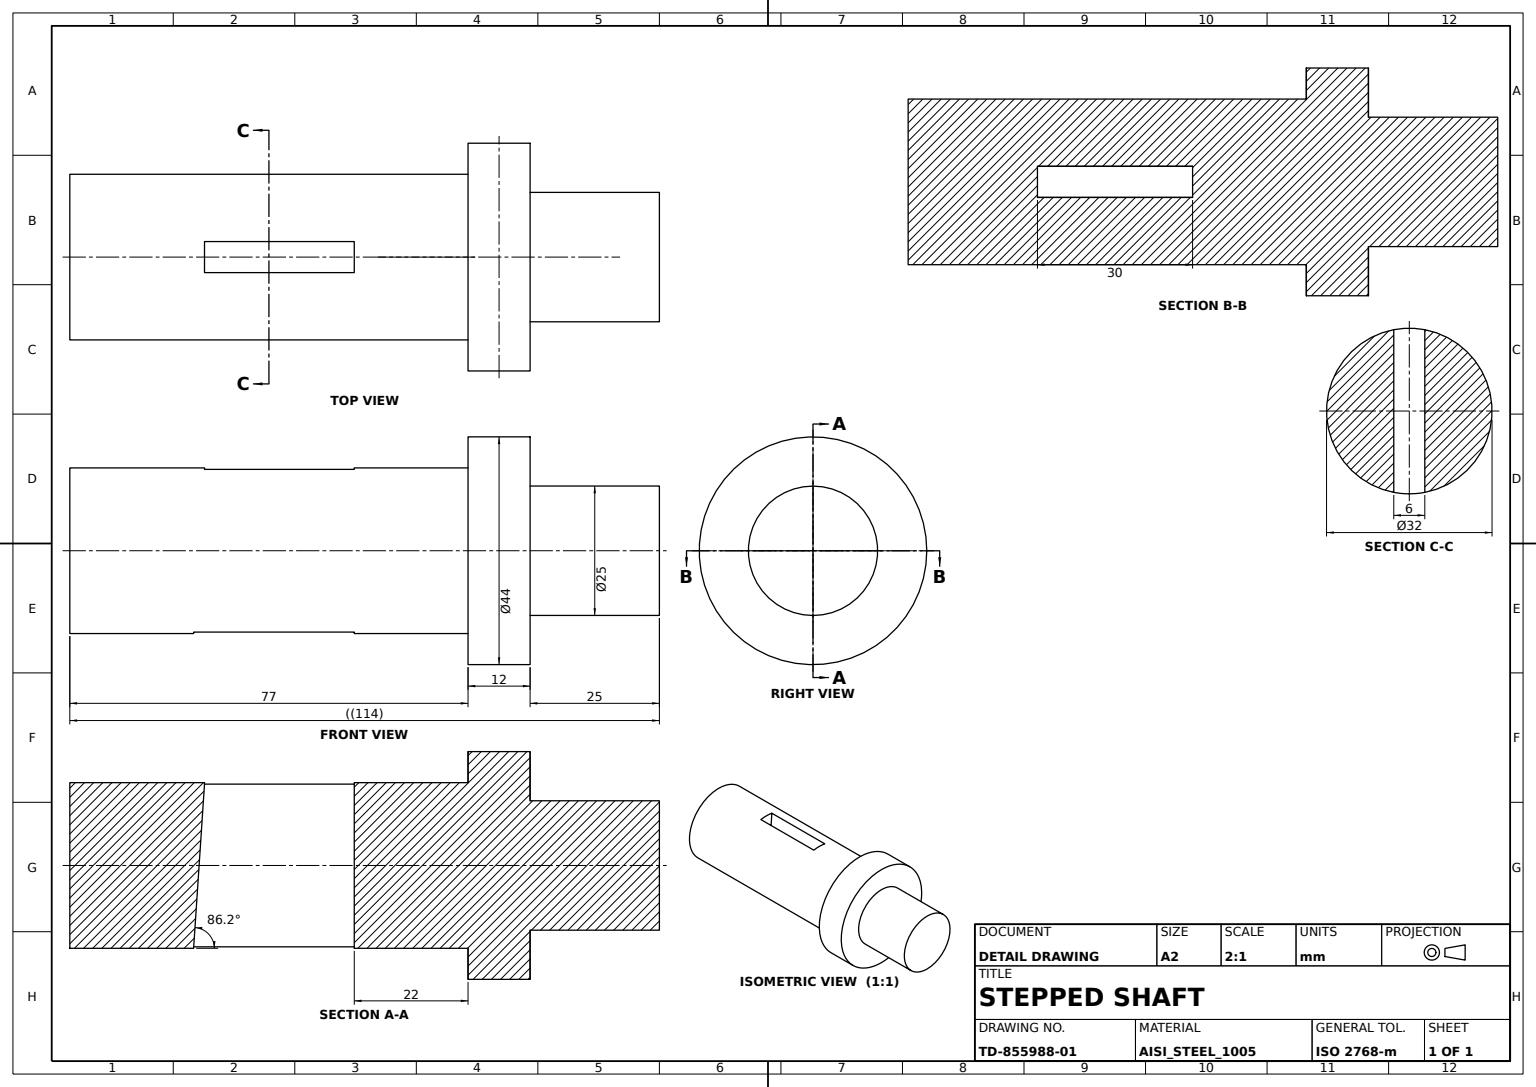
ISO-10303-21;
HEADER;
FILE_DESCRIPTION((''),'2;1');
FILE_NAME('','',(''),(''),'','','');
FILE_SCHEMA(('AUTOMOTIVE_DESIGN'));
ENDSEC;
DATA;
#1=APPLICATION_CONTEXT('');
#2=PRODUCT_CONTEXT('',#1,'mechanical');
#3=PRODUCT('','','',(#2));
#4=PRODUCT_DEFINITION_FORMATION('','',#3);
#5=PRODUCT_DEFINITION_CONTEXT('',#1,'design');
#6=PRODUCT_DEFINITION('','',#4,#5);
#7=PRODUCT_DEFINITION_SHAPE('','',#6);
#8=(LENGTH_UNIT()NAMED_UNIT(*)SI_UNIT(.MILLI.,.METRE.));
#9=(NAMED_UNIT(*)PLANE_ANGLE_UNIT()SI_UNIT($,.RADIAN.));
#10=(NAMED_UNIT(*)SI_UNIT($,.STERADIAN.)SOLID_ANGLE_UNIT());
#11=UNCERTAINTY_MEASURE_WITH_UNIT(LENGTH_MEASURE(0.005),#8,'distance_accuracy_value','');
#12=(GEOMETRIC_REPRESENTATION_CONTEXT(3)GLOBAL_UNCERTAINTY_ASSIGNED_CONTEXT((#11))GLOBAL_UNIT_ASSIGNED_CONTEXT((#8,#9,#10))REPRESENTATION_CONTEXT('',''));
#13=CARTESIAN_POINT('',(16.,0.,-77.));
#14=VERTEX_POINT('',#13);
#15=CARTESIAN_POINT('',(0.,0.,-77.));
#16=DIRECTION('',(0.,0.,-1.));
#17=DIRECTION('',(1.,0.,0.));
#18=AXIS2_PLACEMENT_3D('',#15,#16,#17);
#19=CIRCLE('',#18,16.);
#20=EDGE_CURVE('',#14,#14,#19,.T.);
#21=ORIENTED_EDGE('',*,*,#20,.T.);
#22=EDGE_LOOP('',(#21));
#23=FACE_BOUND('',#22,.T.);
#24=DIRECTION('',(-1.,0.,0.));
#25=AXIS2_PLACEMENT_3D('',#15,#16,#24);
#26=PLANE('',#25);
#27=ADVANCED_FACE('',(#23),#26,.T.);
#28=CARTESIAN_POINT('',(0.,22.,12.));
#29=VERTEX_POINT('',#28);
#30=CARTESIAN_POINT('',(0.,0.,12.));
#31=DIRECTION('',(0.,0.,1.));
#32=DIRECTION('',(0.,1.,0.));
#33=AXIS2_PLACEMENT_3D('',#30,#31,#32);
#34=CIRCLE('',#33,22.);
#35=EDGE_CURVE('',#29,#29,#34,.T.);
#36=ORIENTED_EDGE('',*,*,#35,.T.);
#37=EDGE_LOOP('',(#36));
#38=FACE_BOUND('',#37,.T.);
#39=CARTESIAN_POINT('',(12.5,0.,12.));
#40=VERTEX_POINT('',#39);
#41=AXIS2_PLACEMENT_3D('',#30,#31,#17);
#42=CIRCLE('',#41,12.5);
#43=EDGE_CURVE('',#40,#40,#42,.T.);
#44=ORIENTED_EDGE('',*,*,#43,.F.);
#45=EDGE_LOOP('',(#44));
#46=FACE_BOUND('',#45,.T.);
#47=PLANE('',#41);
#48=ADVANCED_FACE('',(#38,#46),#47,.T.);
#49=CARTESIAN_POINT('',(16.,0.,0.));
#50=VERTEX_POINT('',#49);
#51=CARTESIAN_POINT('',(0.,0.,0.));
#52=AXIS2_PLACEMENT_3D('',#51,#16,#17);
#53=CIRCLE('',#52,16.);
#54=EDGE_CURVE('',#50,#50,#53,.T.);
#55=ORIENTED_EDGE('',*,*,#54,.F.);
#56=EDGE_LOOP('',(#55));
#57=FACE_BOUND('',#56,.T.);
#58=CARTESIAN_POINT('',(0.,22.,0.));
#59=VERTEX_POINT('',#58);
#60=AXIS2_PLACEMENT_3D('',#51,#31,#32);
#61=CIRCLE('',#60,22.);
#62=EDGE_CURVE('',#59,#59,#61,.T.);
#63=ORIENTED_EDGE('',*,*,#62,.F.);
#64=EDGE_LOOP('',(#63));
#65=FACE_BOUND('',#64,.T.);
#66=AXIS2_PLACEMENT_3D('',#51,#31,#17);
#67=PLANE('',#66);
#68=ADVANCED_FACE('',(#57,#65),#67,.F.);
#69=ORIENTED_EDGE('',*,*,#62,.T.);
#70=EDGE_LOOP('',(#69));
#71=FACE_BOUND('',#70,.T.);
#72=ORIENTED_EDGE('',*,*,#35,.F.);
#73=EDGE_LOOP('',(#72));
#74=FACE_BOUND('',#73,.T.);
#75=AXIS2_PLACEMENT_3D('',#30,#16,#24);
#76=CYLINDRICAL_SURFACE('',#75,22.);
#77=ADVANCED_FACE('',(#71,#74),#76,.T.);
#78=CARTESIAN_POINT('',(-15.716234,3.,-50.956129));
#79=VERTEX_POINT('',#78);
#80=CARTESIAN_POINT('',(15.716234,3.,-53.043871));
#81=VERTEX_POINT('',#80);
#82=CARTESIAN_POINT('',(24.,3.,-53.594078));
#83=DIRECTION('',(-0.997801468,0.,0.0662739));
#84=VECTOR('',#83,1000.);
#85=LINE('',#82,#84);
#86=EDGE_CURVE('',#79,#81,#85,.F.);
#87=ORIENTED_EDGE('',*,*,#86,.T.);
#88=CARTESIAN_POINT('',(15.716234,3.,-22.));
#89=VERTEX_POINT('',#88);
#90=CARTESIAN_POINT('',(15.716234,3.,-77.));
#91=VECTOR('',#31,1000.);
#92=LINE('',#90,#91);
#93=EDGE_CURVE('',#81,#89,#92,.T.);
#94=ORIENTED_EDGE('',*,*,#93,.T.);
#95=CARTESIAN_POINT('',(-15.716234,3.,-22.));
#96=VERTEX_POINT('',#95);
#97=CARTESIAN_POINT('',(-50.675228,3.,-22.));
#98=VECTOR('',#17,1000.);
#99=LINE('',#97,#98);
#100=EDGE_CURVE('',#89,#96,#99,.F.);
#101=ORIENTED_EDGE('',*,*,#100,.T.);
#102=CARTESIAN_POINT('',(-15.716234,3.,-77.));
#103=LINE('',#102,#91);
#104=EDGE_CURVE('',#96,#79,#103,.F.);
#105=ORIENTED_EDGE('',*,*,#104,.T.);
#106=EDGE_LOOP('',(#87,#94,#101,#105));
#107=FACE_BOUND('',#106,.T.);
#108=CARTESIAN_POINT('',(0.,3.,0.));
#109=DIRECTION('',(0.,-1.,0.));
#110=AXIS2_PLACEMENT_3D('',#108,#109,#16);
#111=PLANE('',#110);
#112=ADVANCED_FACE('',(#107),#111,.T.);
#113=CARTESIAN_POINT('',(15.716234,-3.,-22.));
#114=VERTEX_POINT('',#113);
#115=CARTESIAN_POINT('',(-15.716234,-3.,-22.));
#116=VERTEX_POINT('',#115);
#117=CARTESIAN_POINT('',(-50.675228,-3.,-22.));
#118=LINE('',#117,#98);
#119=EDGE_CURVE('',#114,#116,#118,.F.);
#120=ORIENTED_EDGE('',*,*,#119,.F.);
#121=CARTESIAN_POINT('',(15.716234,-3.,-53.043871));
#122=VERTEX_POINT('',#121);
#123=CARTESIAN_POINT('',(15.716234,-3.,-77.));
#124=LINE('',#123,#91);
#125=EDGE_CURVE('',#122,#114,#124,.T.);
#126=ORIENTED_EDGE('',*,*,#125,.F.);
#127=CARTESIAN_POINT('',(-15.716234,-3.,-50.956129));
#128=VERTEX_POINT('',#127);
#129=CARTESIAN_POINT('',(24.,-3.,-53.594078));
#130=LINE('',#129,#84);
#131=EDGE_CURVE('',#128,#122,#130,.F.);
#132=ORIENTED_EDGE('',*,*,#131,.F.);
#133=CARTESIAN_POINT('',(-15.716234,-3.,-77.));
#134=LINE('',#133,#91);
#135=EDGE_CURVE('',#116,#128,#134,.F.);
#136=ORIENTED_EDGE('',*,*,#135,.F.);
#137=EDGE_LOOP('',(#120,#126,#132,#136));
#138=FACE_BOUND('',#137,.T.);
#139=CARTESIAN_POINT('',(0.,-3.,0.));
#140=AXIS2_PLACEMENT_3D('',#139,#109,#16);
#141=PLANE('',#140);
#142=ADVANCED_FACE('',(#138),#141,.F.);
#143=CARTESIAN_POINT('',(12.5,0.,37.));
#144=VERTEX_POINT('',#143);
#145=CARTESIAN_POINT('',(0.,0.,37.));
#146=AXIS2_PLACEMENT_3D('',#145,#31,#17);
#147=CIRCLE('',#146,12.5);
#148=EDGE_CURVE('',#144,#144,#147,.T.);
#149=ORIENTED_EDGE('',*,*,#148,.T.);
#150=EDGE_LOOP('',(#149));
#151=FACE_BOUND('',#150,.T.);
#152=PLANE('',#146);
#153=ADVANCED_FACE('',(#151),#152,.T.);
#154=ORIENTED_EDGE('',*,*,#131,.T.);
#155=CARTESIAN_POINT('',(0.,0.,-52.));
#156=DIRECTION('',(0.0662739,0.,0.997801468));
#157=AXIS2_PLACEMENT_3D('',#155,#156,#83);
#158=ELLIPSE('',#157,16.035254,16.);
#159=EDGE_CURVE('',#122,#81,#158,.T.);
#160=ORIENTED_EDGE('',*,*,#159,.T.);
#161=ORIENTED_EDGE('',*,*,#86,.F.);
#162=EDGE_CURVE('',#79,#128,#158,.T.);
#163=ORIENTED_EDGE('',*,*,#162,.T.);
#164=EDGE_LOOP('',(#154,#160,#161,#163));
#165=FACE_BOUND('',#164,.T.);
#166=DIRECTION('',(0.997801468,0.,-0.0662739));
#167=AXIS2_PLACEMENT_3D('',#82,#156,#166);
#168=PLANE('',#167);
#169=ADVANCED_FACE('',(#165),#168,.T.);
#170=CARTESIAN_POINT('',(0.,0.,-22.));
#171=AXIS2_PLACEMENT_3D('',#170,#16,#24);
#172=CIRCLE('',#171,16.);
#173=EDGE_CURVE('',#116,#96,#172,.T.);
#174=ORIENTED_EDGE('',*,*,#173,.T.);
#175=ORIENTED_EDGE('',*,*,#100,.F.);
#176=EDGE_CURVE('',#89,#114,#172,.T.);
#177=ORIENTED_EDGE('',*,*,#176,.T.);
#178=ORIENTED_EDGE('',*,*,#119,.T.);
#179=EDGE_LOOP('',(#174,#175,#177,#178));
#180=FACE_BOUND('',#179,.T.);
#181=AXIS2_PLACEMENT_3D('',#97,#16,#24);
#182=PLANE('',#181);
#183=ADVANCED_FACE('',(#180),#182,.T.);
#184=ORIENTED_EDGE('',*,*,#125,.T.);
#185=ORIENTED_EDGE('',*,*,#176,.F.);
#186=ORIENTED_EDGE('',*,*,#93,.F.);
#187=ORIENTED_EDGE('',*,*,#159,.F.);
#188=EDGE_LOOP('',(#184,#185,#186,#187));
#189=FACE_BOUND('',#188,.T.);
#190=ORIENTED_EDGE('',*,*,#20,.F.);
#191=EDGE_LOOP('',(#190));
#192=FACE_BOUND('',#191,.T.);
#193=ORIENTED_EDGE('',*,*,#173,.F.);
#194=ORIENTED_EDGE('',*,*,#135,.T.);
#195=ORIENTED_EDGE('',*,*,#162,.F.);
#196=ORIENTED_EDGE('',*,*,#104,.F.);
#197=EDGE_LOOP('',(#193,#194,#195,#196));
#198=FACE_BOUND('',#197,.T.);
#199=ORIENTED_EDGE('',*,*,#54,.T.);
#200=EDGE_LOOP('',(#199));
#201=FACE_BOUND('',#200,.T.);
#202=AXIS2_PLACEMENT_3D('',#15,#31,#17);
#203=CYLINDRICAL_SURFACE('',#202,16.);
#204=ADVANCED_FACE('',(#189,#192,#198,#201),#203,.T.);
#205=ORIENTED_EDGE('',*,*,#43,.T.);
#206=EDGE_LOOP('',(#205));
#207=FACE_BOUND('',#206,.T.);
#208=ORIENTED_EDGE('',*,*,#148,.F.);
#209=EDGE_LOOP('',(#208));
#210=FACE_BOUND('',#209,.T.);
#211=AXIS2_PLACEMENT_3D('',#145,#16,#24);
#212=CYLINDRICAL_SURFACE('',#211,12.5);
#213=ADVANCED_FACE('',(#207,#210),#212,.T.);
#214=CLOSED_SHELL('',(#27,#48,#68,#77,#112,#142,#153,#169,#183,#204,#213));
#215=MANIFOLD_SOLID_BREP('',#214);
#216=ADVANCED_BREP_SHAPE_REPRESENTATION('',(#215),#12);
#217=SHAPE_DEFINITION_REPRESENTATION(#7,#216);
ENDSEC;
END-ISO-10303-21;
